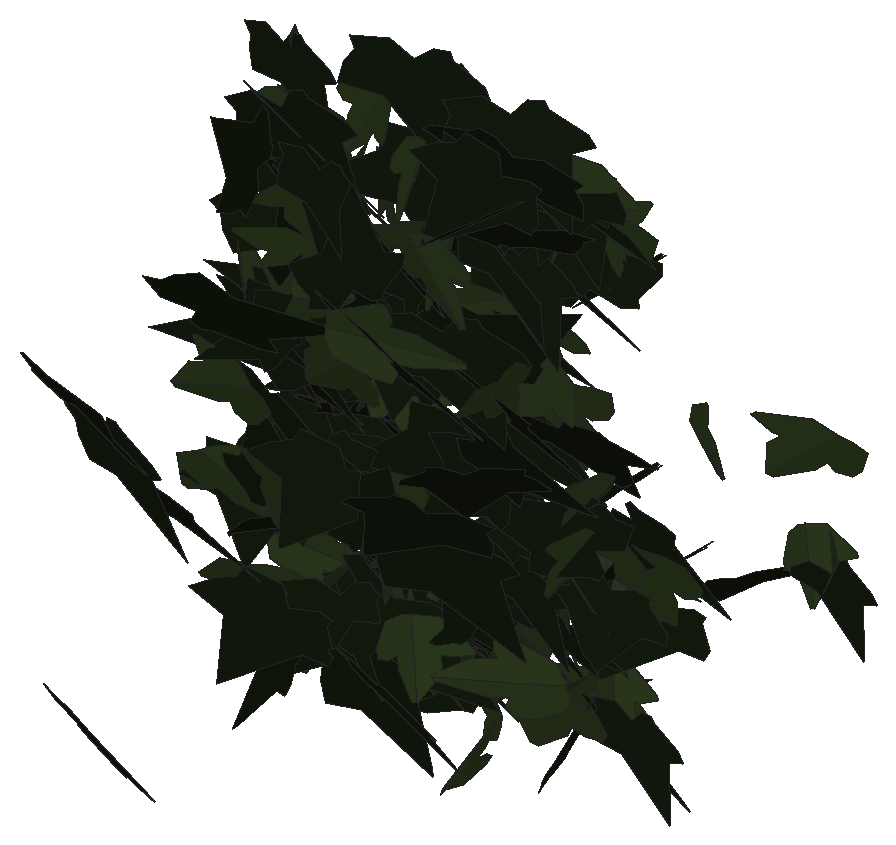
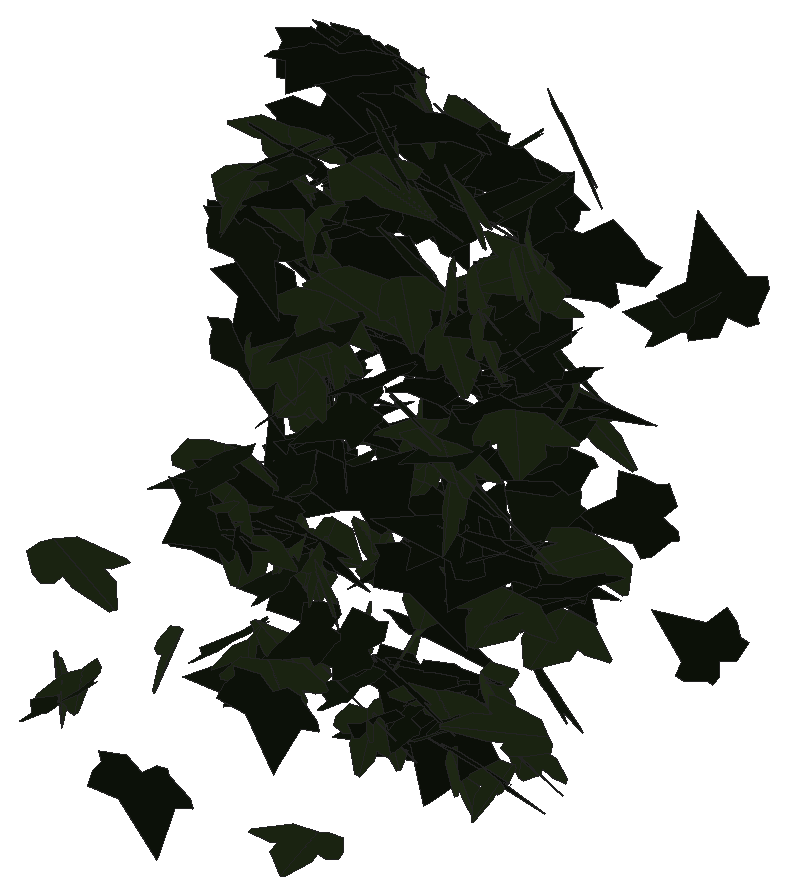
# SketchUp Ruby script. Lengths in millimetres.
U = 1.mm
M = Sketchup.active_model
def pt(a) = Geom::Point3d.new(a.map { |v| v * U })
def face(e, loops, mat)
  f = e.add_face(loops[0].map { |a| pt(a) })
  loops[1..].each { |l| e.add_face(l.map { |a| pt(a) }).erase! }
  f.material = f.back_material = mat if mat
  f
end
# faces: each face lists its corners as indices into pts; further lists are holes
def faces(e, pts, list, mat = nil) = list.each { |f| face(e, (f[0].is_a?(Array) ? f : [f]).map { |l| l.map { |i| pts[i] } }, mat) }
# xy, xz, yz: faces in a plane at the given z, y or x. An outline is a flat list of corners, or four numbers for a rectangle; further outlines are holes
def ring(l) = l.size == 4 ? [[l[0], l[1]], [l[2], l[1]], [l[2], l[3]], [l[0], l[3]]] : l.each_slice(2).to_a
def flat(e, list, mat, &to3) = list.each { |f| face(e, (f[0].is_a?(Array) ? f : [f]).map { |l| ring(l).map { |u, v| to3.(u, v) } }, mat) }
def xy(e, z, list, mat = nil) = flat(e, list, mat) { |x, y| [x, y, z] }
def xz(e, y, list, mat = nil) = flat(e, list, mat) { |x, z| [x, y, z] }
def yz(e, x, list, mat = nil) = flat(e, list, mat) { |y, z| [x, y, z] }
def lines(e, pts, list) = list.each { |a, b| e.add_line(pt(pts[a]), pt(pts[b])) }
# prism: a flat outline (further loops are holes) pulled along v
def prism(e, loops, v, mat = nil)
  f = face(e, loops, mat); d = Geom::Vector3d.new(v.map { |x| x * U })
  f.pushpull(f.normal.samedirection?(d) ? d.length : -d.length)
end
def box(e, o, s, mat = nil) = prism(e, [[o, [o[0] + s[0], o[1], o[2]], [o[0] + s[0], o[1] + s[1], o[2]], [o[0], o[1] + s[1], o[2]]]], [0, 0, s[2]], mat)
def at(x, y, z, deg = 0) = Geom::Transformation.translation(pt([x, y, z])) * Geom::Transformation.rotation(ORIGIN, Z_AXIS, deg.degrees)
def axes(o, x, y, z) = Geom::Transformation.new([*x, 0, *y, 0, *z, 0, *pt(o).to_a, 1])
def part(name) = M.definitions.add(name)
# library, detail: a bought-in or finely detailed component or shape, given as its bounding box
def library(name, o, s) = part(name).tap { |d| box(d.entities, o, s) }
def detail(e, o, s) = box(e.add_group.entities, o, s)
def put(e, d, t, mat = nil) = e.add_instance(d, t).tap { |i| i.material = mat if mat }
def group(e, t, mat = nil) = e.add_group.tap { |g| g.transformation = t; g.material = mat if mat }.entities
root = M.entities
M.materials.add("efeu1").color = [18, 25, 13]
M.materials.add("efeu2").color = [43, 57, 29]
c1 = part("ivyleaf_10")
p = [[0,12.8,-0.8],[-1.5,51.3,-10.9],[-4.9,51,-11.6],[-13.6,26.5,-7.3],[-13.2,15.9,-4.6],[-21.1,19.3,-7.2],
  [-29.5,16.3,-8.3],[-29.2,8.3,-6.2],[-19.7,-9.8,0.5],[-7.6,-13,4],[1,-12.2,5.8],[-0.4,51.1,-11.1],
  [-1.5,51.1,-10.9],[1,-12.4,5.9],[16.9,-12.4,3.5],[35.1,9.1,-5.1],[35,12.9,-6.1],[20.5,16.4,-4.9],
  [15.8,15,-3.8],[15.3,27.6,-7.1],[12.8,31.3,-7.8]]
faces(c1.entities,p,[[0,1,2,3,4,5,6,7,8,9,10],[11,12,0,13,14,15,16,17,18,19,20]],"efeu2")
c2 = part("ivyleaf_9")
p = [[39.1,54.8,31.7],[34.5,51.8,30.2],[-5.3,25.2,17.3],[-17.9,28.3,20.9],[-21.6,21.7,17],[-20.2,4.3,5.3],
  [-22.9,-0.3,2.5],[-17.1,-4,-0.6],[-2,-2.1,-1.2],[-0.7,-15.4,-10.1],[16.6,-22.3,-16.7],[21.1,-15.1,-12.5],
  [32.7,-10.7,-11],[46.1,-1.8,-6.6],[30.8,11.2,3.8]]
faces(c2.entities,p,[[0,1,2,3,4,5,6,7,8,9,10,11,12,13,14]],"efeu1")
put(root,c1,axes([5796.8,665.9,3906.6],[-0.334,1.13497,-0.54632],[0.05256,-0.548,-1.14733],[-2.39672,-0.17018,0.05097]))
put(root,c2,axes([5795.1,740.7,3667.1],[-0.39675,-1.1687,0.01594],[0.00619,-0.01677,-1.18713],[2.22447,-0.2084,0.00615]))
put(root,c2,axes([5800.6,675.8,3671.1],[-0.80713,-1.1442,0.03662],[-0.02069,-0.03502,-1.22027],[2.17866,-0.42423,0.00198]))
put(root,c2,axes([5787.4,726.4,3996.3],[0.43543,-1.15832,-0.36483],[-0.12512,0.35889,-1.18069],[2.30789,0.238,0.00482]))
put(root,c2,axes([5772.2,444.1,3486.4],[0.67007,-0.77947,0.88639],[0.78469,-0.7855,-0.85452],[2.10497,0.54095,0.03639]))
put(root,c1,axes([5771.8,776.8,3538.8],[0.44711,0.17688,1.12767],[1.75643,0.6481,-0.29392],[-1.27844,0.95227,-0.00942]))
put(root,c1,axes([5809.5,773.5,3472.8],[0.06326,0.95136,0.64808],[-0.18696,0.64833,-0.94669],[-2.18284,-0.02796,0.09987]))
put(root,c2,axes([5787.2,702.7,3951.1],[0.40232,-0.971,-0.71315],[0.22026,0.73707,-0.96926],[2.28229,0.10003,0.21925]))
put(root,c2,axes([5775.5,541.7,3704.5],[1.95629,-0.57689,0.28594],[0.45149,-0.16143,-1.17847],[1.1392,1.05464,-0.02398]))
put(root,c1,axes([5798.9,740.6,3498.4],[1.98905,-0.35637,0.40377],[0.7281,-0.12915,-1.1042],[0.7214,1.11293,0.00116]))
put(root,c1,axes([5791.5,633.5,3697],[-1.72743,-0.13985,-0.81354],[1.56922,-0.09528,-0.90351],[0.07576,-1.21515,0.16447]))
put(root,c1,axes([5857.2,580.1,3829.6],[-1.23871,0.16423,1.01664],[-1.941,0.06405,-0.66327],[-0.2719,-1.20543,0.10327]))
put(root,c1,axes([5827.5,723.1,3881.6],[-1.58643,-0.91265,0.03042],[0.20371,-0.13855,-1.22394],[1.72594,-0.82253,0.17242]))
put(root,c1,axes([5828.9,713,4076.7],[0.14606,-1.24687,-0.06836],[-0.00446,0.06835,-1.24923],[2.3766,0.07676,0.00186]))
put(root,c2,axes([5792.4,682.7,3851.4],[0.87222,-1.11921,0.29812],[0.25648,-0.2669,-1.20919],[2.18938,0.47715,0.02289]))
put(root,c1,axes([5818.1,758.2,3676.9],[-2.00969,-0.4188,-0.37007],[0.70108,0.07338,-1.13415],[0.7999,-1.11651,0.06427]))
put(root,c2,axes([5782.9,724.2,3988.2],[1.81822,-0.91922,0.37954],[0.50747,-0.27026,-1.32573],[1.82341,0.99182,-0.0095]))
put(root,c1,axes([5811.7,720.4,4118.6],[0.4129,-0.40986,1.14936],[1.34286,-0.91031,-0.45779],[1.89478,0.73446,0.07398]))
put(root,c2,axes([5854.6,731.7,3494.6],[-1.93697,0.40526,-0.37422],[0.57062,-0.25279,-1.08916],[-0.88121,-1.05449,0.11728]))
put(root,c2,axes([5807,693.3,3749.7],[0.35081,-1.06405,0.72876],[0.51452,-0.68793,-1.07282],[2.39999,0.30302,0.12347]))
put(root,c2,axes([5877.2,707.8,3857.9],[-0.54542,0.13541,1.18924],[-2.20259,-0.34334,-0.23979],[0.5812,-1.17411,0.20727]))
put(root,c2,axes([5868.5,782.2,3482.6],[-2.10767,0.22953,0.00729],[-0.07182,-0.14646,-1.12084],[-0.43113,-1.09773,0.15107]))
put(root,c2,axes([5809.5,381.8,3879.2],[2.30917,-0.69271,-0.54022],[0.98007,-0.18545,1.39436],[-1.3545,-1.31513,0.08793]))
put(root,c1,axes([5839.9,635,3591.3],[-2.1649,-0.24436,-0.30591],[0.56292,0.07954,-1.16336],[0.48823,-1.17523,-0.01513]))
put(root,c2,axes([5813.5,656.2,3828.8],[2.30353,-0.22878,0.07764],[0.14384,-0.0182,-1.23177],[0.43673,1.2127,-0.00384]))
put(root,c1,axes([5852.9,735.5,3552.3],[0.32746,-1.13453,0.29816],[0.02511,-0.29946,-1.14709],[2.23242,0.16978,-0.03083]))
put(root,c2,axes([5869.6,710.7,3988],[-1.9285,0.57898,-0.38317],[0.62719,-0.1956,-1.16703],[-1.16305,-1.06552,0.00602]))
put(root,c2,axes([5838.9,739.4,3723.2],[-0.4965,-1.17157,0.083],[0.05703,-0.09163,-1.19926],[2.23458,-0.25797,0.04905]))
put(root,c2,axes([5884.1,729.3,3790.2],[-1.72681,0.78913,0.0762],[-0.10023,0.05556,-1.20245],[-1.50552,-0.90882,-0.00735]))
put(root,c2,axes([5898.5,634.2,3865.5],[-1.72162,-0.08563,0.9191],[-1.74533,-0.06342,-0.90849],[0.20039,-1.28802,-0.01637]))
put(root,c1,axes([5859.5,785.6,3473.3],[0.10728,-1.14994,-0.01867],[-0.02692,0.01799,-1.15125],[2.18869,0.05659,-0.01325]))
put(root,c2,axes([5832.4,683.2,4146.7],[0.49684,-1.24339,0.04769],[0.00153,-0.04856,-1.27046],[2.36815,0.2609,-0.00919]))
put(root,c2,axes([5858.2,634.3,3662.5],[0.869,1.05762,0.23913],[0.22543,0.20927,-1.1517],[-2.05132,0.47103,-0.02526]))
put(root,c2,axes([5848.7,737.8,3734.2],[1.83436,0.70001,-0.10289],[-0.19701,-0.03249,-1.19071],[-1.33208,0.96876,0.03442]))
put(root,c1,axes([5820.4,705.7,4068.9],[1.68517,-0.30802,0.84232],[1.70439,0.23909,-0.85395],[0.0931,1.19848,0.38684]))
put(root,c2,axes([5827.7,716.4,4018.2],[1.91441,-0.73274,-0.00047],[0.10005,0.07297,-1.24122],[1.39096,1.00324,0.08993]))
put(root,c1,axes([5869,724.6,3991.1],[-0.11923,-1.23346,0.02125],[-0.00272,-0.0212,-1.23505],[2.34787,-0.06266,-0.00035]))
put(root,c2,axes([5872.6,629.5,3516.1],[-1.50831,0.48977,-0.69106],[1.10614,-0.374,-0.93158],[-1.17267,-0.98273,0.01012]))
put(root,c2,axes([5891.4,655.9,4009.7],[1.05856,0.02583,-1.1473],[-2.18322,-0.0237,-0.55665],[-0.06204,1.2748,0.0129]))
put(root,c2,axes([5836.2,698.7,4045.9],[1.40072,-1.00791,0.08638],[0.06612,-0.08157,-1.24786],[1.92416,0.73653,-0.02]))
put(root,c2,axes([5878.6,753.6,3737.5],[-2.02455,-0.5304,-0.16639],[0.35453,-0.00163,-1.1857],[0.99679,-1.07669,0.08376]))
put(root,c2,axes([5884.7,603.5,3706.4],[1.41341,-0.34365,0.93272],[-0.72823,0.97574,0.66417],[-1.74603,-0.68515,0.47803]))
put(root,c2,axes([5911.2,584.2,3910.9],[-1.74842,0.80914,-0.13427],[0.16788,-0.10297,-1.22405],[-1.55195,-0.92271,0.01886]))
put(root,c2,axes([5879.8,767.5,3498.2],[1.9356,0.42232,-0.42053],[-0.77024,-0.12119,-1.10048],[-0.83266,1.09384,0.04043]))
put(root,c1,axes([5892,703.1,4030.4],[-0.16776,-1.25739,-0.08719],[0.00034,0.08739,-1.26047],[2.39882,-0.08795,-0.00592]))
put(root,c1,axes([5891.6,654.6,4022],[-1.43648,-1.00158,-0.09615],[0.16857,0.05359,-1.25354],[1.90753,-0.75898,0.03837]))
put(root,c1,axes([5908.5,626.5,3973.2],[-2.07098,-0.46036,0.41268],[-0.62058,-0.28242,-1.17483],[0.99971,-1.12899,0.12561]))
put(root,c2,axes([5856,742.1,3727.9],[1.0907,-0.03688,1.05806],[1.77323,0.58893,-0.48412],[-0.95687,1.04933,0.3089]))
put(root,c1,axes([5892.9,754.6,3781.3],[0.09887,-1.02424,-0.60939],[0.21943,0.61142,-1.01784],[2.25763,-0.01457,0.12562]))
put(root,c2,axes([5859.6,646.3,3863],[1.1828,-1.04,0.1457],[0.1814,-0.11274,-1.21131],[1.9904,0.62829,0.02381]))
put(root,c2,axes([5882.4,784.9,3505.2],[-0.6573,-1.0132,0.42149],[0.09429,-0.45582,-1.05512],[2.08639,-0.2986,0.18047]))
put(root,c2,axes([5850.2,635.9,4109.5],[1.8345,-0.93429,0.32696],[0.44831,-0.22675,-1.34239],[1.82975,0.99227,0.0011]))
put(root,c2,axes([5858,378.8,3863.4],[1.06925,-1.36745,0.26542],[0.19892,-0.244,-1.47836],[2.64363,0.57144,0.00389]))
put(root,c1,axes([5894.3,771,3536.3],[2.14849,0.22971,-0.21732],[-0.39215,-0.07681,-1.15153],[-0.45653,1.14704,-0.03359]))
put(root,c2,axes([5935.6,506.4,4129.3],[-0.90013,0.22933,-1.41585],[-2.38064,0.66355,0.52532],[1.33573,1.33717,-0.01786]))
put(root,c1,axes([5881.6,1018.8,3474.9],[1.36929,0.79738,0.35485],[0.37302,0.30052,-1.07268],[-1.61863,0.7438,0.05299]))
put(root,c2,axes([5914.3,579.1,3603.7],[-2.15669,-0.46089,-0.14815],[0.25504,0.06373,-1.2233],[0.88536,-1.14106,-0.00849]))
put(root,c2,axes([5877.4,732.9,3857.4],[1.67334,-0.80287,-0.18138],[-0.19283,0.15781,-1.18969],[1.55461,0.88376,0.04766]))
put(root,c2,axes([5910.5,758,3529.7],[-1.01703,-0.93945,0.40443],[-0.30539,-0.37364,-1.07997],[1.9225,-0.55634,0.0424]))
put(root,c1,axes([5903.7,747.3,3834.8],[2.27086,-0.16716,-0.00538],[-0.0128,-0.00925,-1.20479],[0.31805,1.19315,-0.0101]))
put(root,c1,axes([5921,722.2,3955.4],[-0.74148,-1.17178,0.09335],[0.02893,-0.10336,-1.23396],[2.23702,-0.38706,0.0469]))
put(root,c2,axes([5903.8,657.5,4026.3],[-0.28963,-1.04921,0.79209],[-0.04706,-0.79495,-1.05775],[2.50155,-0.13643,0.07181]))
put(root,c2,axes([5939.1,745.7,3683.1],[0.36559,1.05919,-0.53623],[-0.37314,-0.50744,-1.07256],[-2.22844,0.25874,0.09163]))
put(root,c2,axes([5887.8,612.3,4125.7],[-0.71202,-0.29937,-1.24944],[2.25992,0.41639,-0.45532],[0.93379,-1.23599,0.14924]))
put(root,c2,axes([5939.4,744,3549.2],[-1.97214,-0.52652,0.05533],[-0.0399,-0.0807,-1.16064],[1.00681,-1.03456,0.06238]))
put(root,c1,axes([5927.4,746,3664],[-2.18693,-0.30642,-0.11692],[0.2528,-0.04533,-1.1867],[0.57069,-1.15412,0.07765]))
put(root,c2,axes([5875.3,501.7,3952.1],[0.53463,-0.35415,1.26589],[2.33503,-0.39399,-0.38248],[0.89796,1.23538,0.24091]))
put(root,c2,axes([5900.3,747.1,3521.8],[1.42691,-0.88297,0.03543],[0.01785,-0.03851,-1.1582],[1.68172,0.74959,-0.01777]))
put(root,c1,axes([5951.2,535,3772.4],[-1.98349,0.48543,0.45725],[-0.82928,0.14655,-1.14871],[-0.96081,-1.12861,0.04751]))
put(root,c1,axes([5935.5,687.1,4122.8],[1.54118,-0.96446,-0.08158],[-0.10404,0.06063,-1.25934],[1.83918,0.81162,-0.00288]))
put(root,c2,axes([5959.9,730.9,3688.7],[-1.55565,-0.63087,0.84082],[-1.25444,-0.52211,-1.0325],[1.55846,-1.05,0.00822]))
put(root,c2,axes([5918.9,735.8,3736.1],[1.98078,-0.36395,-0.46289],[-0.8344,0.14857,-1.10256],[0.74811,1.12933,-0.00413]))
put(root,c1,axes([5926.5,713.4,4026.2],[0.89529,-1.13561,-0.10487],[0.67342,0.25318,-1.15439],[2.06339,0.41011,0.42225]))
put(root,c2,axes([5974.4,776.5,3458.2],[-0.5602,-0.0008,1.12445],[-2.04946,-0.33441,-0.28213],[0.61608,-1.11319,0.08394]))
put(root,c2,axes([5902.7,641.9,3924.4],[0.48464,-0.04985,1.34194],[2.46138,0.37684,-0.23141],[-0.68809,1.31288,0.11738]))
put(root,c2,axes([5970.4,778.5,3552.3],[-2.02836,0.4474,-0.10971],[0.21814,-0.01027,-1.15534],[-0.84915,-1.07135,-0.03474]))
put(root,c2,axes([5974.5,711.9,3579.9],[-2.1723,-0.06918,0.19169],[-0.36733,0.0169,-1.14314],[0.1245,-1.15725,-0.02815]))
put(root,c2,axes([5946.2,742.1,3535],[1.82326,0.53116,-0.38862],[-0.87864,0.05321,-1.06534],[-0.89273,1.03245,0.25484]))
put(root,c1,axes([5940.6,571,3961.2],[0.00175,-0.48505,-1.13365],[0.82398,1.0616,-0.45388],[2.19734,-0.3977,0.1711]))
put(root,c2,axes([5935.9,639.5,3595.8],[-0.39883,-1.09969,-0.5919],[0.3071,0.5713,-1.11855],[2.35692,-0.26052,0.04559]))
put(root,c2,axes([5989.9,717.6,3842.9],[-1.94961,0.67503,-0.19723],[0.28481,-0.13126,-1.2265],[-1.30777,-1.03491,0.02691]))
put(root,c2,axes([5933.5,781.9,3502],[1.53642,-0.8004,-0.01432],[0.00238,0.02159,-1.1367],[1.52357,0.80712,0.01621]))
put(root,c2,axes([5961.1,696.5,3879.7],[-0.92994,-1.08793,-0.09546],[0.09798,0.08152,-1.19254],[2.07619,-0.49114,0.01352]))
put(root,c1,axes([5974.8,766.5,3488.4],[-0.45545,-1.15253,-0.03923],[0.02595,0.03724,-1.1771],[2.19462,-0.23963,0.00578]))
put(root,c2,axes([5939.7,646.9,3675.7],[0.34383,-0.8034,1.01493],[0.46614,-0.98504,-0.82334],[2.41904,0.30401,0.0144]))
put(root,c1,axes([6004.9,554.6,3915.9],[-1.73918,0.26509,0.79226],[-1.43493,0.24408,-0.95131],[-0.68488,-1.18455,-0.01872]))
put(root,c1,axes([5983.8,790.7,3481.1],[-1.68336,0.68941,0.18401],[-0.31963,0.0837,-1.12083],[-1.31987,-0.89954,0.03674]))
put(root,c1,axes([5986.6,719.4,3989.9],[-0.77755,-1.17096,-0.06937],[0.05362,0.06364,-1.24017],[2.23183,-0.40948,0.00563]))
put(root,c2,axes([5961,583.6,3785.6],[0.08989,-0.99937,-0.91828],[-0.11716,0.91631,-1.0004],[2.58036,0.07642,-0.01343]))
put(root,c1,axes([5969.5,695,3817.3],[1.12076,1.07279,0.10328],[0.09382,0.09076,-1.22379],[-2.04902,0.59094,0.00046]))
put(root,c1,axes([5983.9,699,3556.6],[0.52306,-0.30312,-1.14992],[0.24851,1.18078,-0.28005],[2.2496,-0.05996,0.29831]))
put(root,c2,axes([5966.1,569.1,4105],[0.21019,-1.23066,0.15811],[-0.01356,-0.15936,-1.23542],[2.36141,0.10862,-0.02117]))
put(root,c2,axes([5969.2,656.5,3688.8],[0.89681,-0.53052,-1.0117],[-0.46102,1.0231,-0.64932],[2.12471,0.44592,0.28614]))
put(root,c2,axes([5968.7,712.9,3911],[-1.12934,-0.69771,-0.81354],[1.63779,0.24412,-0.83704],[1.21584,-0.97692,0.37186]))
put(root,c1,axes([5985.4,659,3605.1],[-0.27073,0.89512,-0.75729],[0.10158,-0.75711,-0.90493],[-2.22916,-0.14321,0.05073]))
put(root,c2,axes([6040.5,651.3,4092.1],[-2.08319,0.48971,0.33079],[-0.73068,-0.05992,-1.18167],[-0.85505,-1.14189,0.20387]))
put(root,c2,axes([6012.2,545,3803.8],[-1.89197,-0.72797,-0.00491],[0.00718,0.00316,-1.23214],[1.38548,-0.99411,-0.00033]))
put(root,c2,axes([6031.1,776.6,3508.2],[-1.8215,0.61294,-0.09726],[0.17801,-0.03425,-1.13632],[-1.16765,-0.96139,-0.02152]))
put(root,c1,axes([5999.3,688.9,3721.3],[-2.03344,-0.33034,-0.38585],[0.78882,-0.04749,-1.10703],[0.55884,-1.13498,0.15862]))
put(root,c2,axes([6025.5,747.8,3721.1],[1.41391,-0.51743,0.79441],[-1.25713,0.44148,0.90527],[-1.29433,-0.99403,-0.01146]))
put(root,c2,axes([5997.1,673.4,4191.4],[-1.35894,-0.64221,-0.79349],[1.36033,0.37683,-0.94817],[1.3871,-0.99873,0.15248]))
put(root,c2,axes([6053.6,644.2,3991.5],[-1.5359,0.93613,0.24763],[-0.37252,0.158,-1.23517],[-1.80488,-0.82923,0.04421]))
put(root,c2,axes([5996.8,789.8,3523.6],[0.47054,-1.0883,0.22054],[0.19352,-0.2028,-1.11477],[2.10448,0.26198,0.0532]))
put(root,c2,axes([6055.6,524.2,3772.9],[-0.07097,0.4332,1.25952],[-0.82498,1.18747,-0.42125],[-2.39694,-0.42153,0.10769]))
put(root,c1,axes([6048.4,712.9,4116.5],[1.31907,0.56764,-0.87375],[-1.64029,-0.2774,-0.86386],[-1.11439,1.08021,0.2373]))
put(root,c2,axes([6031.1,611.9,4003.9],[1.37632,-1.07781,0.32059],[-0.21149,0.3108,1.29555],[-2.12963,-0.72742,0.07853]))
put(root,c2,axes([6038.5,697,4158.1],[-1.57234,0.55261,-0.75821],[1.22708,-0.39953,-0.99372],[-1.2972,-1.04775,-0.02098]))
put(root,c2,axes([5999.2,776.2,3564.8],[1.37643,-0.87902,0.24827],[0.40418,-0.14617,-1.13617],[1.69075,0.75054,0.06949]))
put(root,c2,axes([6023.4,727.7,3875],[-0.37138,-1.19943,0.01731],[-0.02021,-0.01581,-1.21518],[2.28291,-0.19526,-0.00794]))
put(root,c2,axes([6063.5,496.4,4048.1],[-1.99499,0.78346,-0.45317],[-0.689,0.27258,1.30866],[1.57876,1.10898,-0.00151]))
put(root,c2,axes([5994.1,577.7,3737.3],[2.16241,-0.15173,0.67227],[1.2595,-0.12169,-1.14593],[0.36618,1.31457,-0.02849]))
put(root,c2,axes([6081.6,668.1,3785.5],[-0.57598,0.68352,0.93082],[-1.00981,0.77237,-0.73968],[-1.95215,-0.6012,0.10799]))
put(root,c2,axes([6086.8,684,4102.4],[-2.05599,0.51894,0.31171],[-0.57094,0.09493,-1.19769],[-1.00071,-1.12034,0.0429]))
put(root,c2,axes([6085.4,617.8,3822.8],[-1.86236,0.66687,0.18267],[-0.30729,0.08741,-1.18403],[-1.27956,-0.9916,0.01848]))
put(root,c2,axes([6026,594.1,3616.6],[0.93251,-0.71755,-1.15566],[-0.30267,1.1897,-0.80611],[2.57117,0.40029,0.32424]))
put(root,c2,axes([6027.2,564.9,3584.4],[-0.85472,-0.2473,-1.12295],[2.05271,0.32732,-0.50343],[0.75863,-1.16429,0.09699]))
put(root,c1,axes([6067.2,656.6,3674.8],[-1.56945,0.76915,0.3218],[-0.45142,0.21749,-1.12766],[-1.52124,-0.85807,0.00263]))
put(root,c1,axes([6092.4,701.7,3952.5],[1.30962,0.32757,-0.9884],[-1.96323,0.05294,-0.70061],[-0.27017,1.20317,0.29993]))
put(root,c1,axes([6070.1,1022.6,3658.1],[-0.95019,0.95392,0.44885],[-0.34547,0.41144,-1.07632],[-1.97647,-0.53052,-0.02766]))
put(root,c1,axes([6064,589.9,4150.1],[1.163,-0.96069,0.51278],[0.52802,-0.43124,-1.13857],[2.00415,0.67111,0.00241]))
put(root,c1,axes([6068.9,703.1,3495.3],[-1.01131,0.89456,0.65066],[0.60354,-0.56835,1.04037],[2.01688,0.61863,0.01493]))
put(root,c1,axes([6079.3,753.9,3625],[0.98036,-1.02657,-0.21563],[-0.13615,0.20529,-1.14823],[1.99176,0.51932,0.02765]))
put(root,c1,axes([6076.2,564,3739.3],[0.15864,-1.21645,0.30468],[0.22518,-0.29636,-1.21561],[2.37601,0.1093,0.09486]))
put(root,c2,axes([6053.1,773.1,3569.3],[1.61064,-0.74689,-0.2137],[-0.33669,0.12243,-1.12846],[1.43967,0.86422,-0.02483]))
put(root,c2,axes([6050.8,706.5,3816.8],[1.79573,-0.81452,-0.23788],[-0.31949,0.16953,-1.24634],[1.58303,0.95818,0.0183]))
put(root,c2,axes([6091.5,1050.2,3493.5],[0.47299,1.10795,-0.11448],[-0.1735,-0.09667,-1.13347],[-2.11276,0.25598,0.06745]))
put(root,c1,axes([6089.6,739.9,3638.5],[-0.49991,1.10482,0.38543],[-0.47999,0.33228,-1.12435],[-2.17463,-0.32732,0.15957]))
put(root,c1,axes([6091,722.3,3899.2],[1.78325,-0.7882,-0.09332],[0.13848,0.22907,-1.20421],[1.50421,0.91332,0.22149]))
put(root,c2,axes([6104,805.2,3483.3],[0.56342,1.10278,0.04301],[-0.00566,0.04532,-1.14173],[-2.1004,0.29569,0.01461]))
put(root,c2,axes([6081.7,714,3725.2],[-0.10336,0.44264,1.33266],[-0.2745,-1.32836,0.43534],[2.65844,-0.11995,0.09676]))
put(root,c1,axes([6088.3,603.1,4056.1],[1.23356,-0.97045,0.48091],[0.5425,-0.38785,-1.16682],[1.98863,0.70778,0.02]))
put(root,c1,axes([6098.8,718.4,3927.9],[-2.27533,0.13285,-0.14595],[0.26178,-0.08177,-1.2011],[-0.26937,-1.20163,0.0656]))
put(root,c2,axes([6081.9,708.9,3927.9],[1.91378,-0.444,-0.55518],[-0.70738,0.49145,-1.06623],[1.1533,1.0382,0.26729]))
put(root,c1,axes([6097.2,549.9,3655.6],[0.97862,1.12279,-0.18676],[-0.14552,-0.17039,-1.23493],[-2.16137,0.51985,-0.00141]))
put(root,c1,axes([6114.3,658.9,3793.7],[0.27969,-0.72313,-0.979],[-0.2398,0.97177,-0.7367],[2.30395,0.18893,0.04217]))
put(root,c2,axes([6092.4,677.9,4125.1],[-0.42243,-1.22239,0.01612],[-0.0033,-0.01607,-1.24238],[2.32666,-0.22196,0.00117]))
put(root,c2,axes([6133.7,746.8,3657.6],[-2.23755,0.08003,-0.01328],[0.02518,-0.00121,-1.1784],[-0.15233,-1.17575,0.00031]))
put(root,c2,axes([6086.1,721.5,3723],[-0.0457,-1.1326,0.44618],[0.28741,-0.44559,-1.12298],[2.29891,0.0332,0.14927]))
put(root,c1,axes([6114.6,790,3501.7],[1.89902,0.50477,-0.25471],[-0.69216,0.17741,-1.07311],[-0.82392,1.01441,0.31442]))
put(root,c2,axes([6072.1,528.1,3595.3],[0.79393,-1.00323,0.78821],[0.88491,-0.6527,-1.07683],[2.26117,0.60768,0.14467]))
put(root,c1,axes([6103.8,753,3487.5],[-0.42973,-1.13162,0.41676],[0.54374,0.36173,1.137],[-2.22978,0.3063,0.19694]))
put(root,c1,axes([6116.5,715.5,4023.4],[-0.04316,-0.9765,0.74349],[0.69365,-0.71543,-0.92853],[2.23047,0.20359,0.30315]))
put(root,c1,axes([6124.6,741,3656.2],[-1.3214,0.94249,0.13022],[-0.09304,0.12565,-1.1701],[-1.80839,-0.69515,-0.03495]))
put(root,c1,axes([6120.9,730.1,3840.4],[-1.81486,0.71123,-0.27459],[0.3724,-0.19668,-1.18895],[-1.40238,-0.97264,0.03963]))
put(root,c2,axes([6108.7,646.3,3694.1],[-0.01279,-0.69302,-1.08896],[0.0599,1.08856,-0.69296],[2.45588,-0.03016,0.01123]))
put(root,c2,axes([6134.5,612.9,3814.3],[-0.76936,-0.74245,0.89804],[-0.79987,-0.79367,-0.84533],[2.06835,-0.58309,0.00714]))
put(root,c1,axes([6143.3,729.2,3854],[-1.5297,-0.85619,0.34099],[-0.30802,-0.31429,-1.17063],[1.72672,-0.81456,0.09326]))
put(root,c2,axes([6104.1,778.1,3618.2],[0.77975,-1.08647,0.0558],[0.0233,-0.05502,-1.16113],[2.07036,0.40981,-0.00795]))
put(root,c1,axes([6128.1,669,3615.3],[-0.41808,-0.9108,-0.79876],[0.52457,0.75292,-0.93433],[2.24513,-0.34552,0.06956]))
put(root,c2,axes([6114,649.8,3692.9],[1.91054,0.61352,0.20599],[0.27295,0.15982,-1.17493],[-1.20109,1.01223,0.06066]))
put(root,c2,axes([6084.6,477.4,4012.3],[1.49461,-0.97461,0.83994],[1.07165,-0.62446,-1.25104],[2.20173,0.96554,0.03873]))
put(root,c2,axes([6118.1,691.1,3826.7],[1.07179,-0.72783,-0.80416],[-0.55086,0.77239,-0.90177],[1.98941,0.60599,0.18354]))
put(root,c1,axes([6121.3,533.1,4088.6],[-1.53731,0.54525,-0.78349],[0.89503,-0.66584,-0.94821],[-1.5809,-0.90718,0.22505]))
put(root,c2,axes([6105.1,626.9,3933.3],[-0.71844,-0.04199,1.26437],[2.3327,-0.33884,0.35469],[0.59614,1.27527,0.13587]))
put(root,c1,axes([6103.5,449.7,4026.3],[0.02648,0.03971,1.26397],[1.89655,0.77789,-0.03541],[-1.48177,0.99634,-0.02273]))
put(root,c2,axes([6174.8,762.7,3643.5],[-2.02883,-0.31545,0.39903],[-0.72918,-0.11152,-1.1117],[0.63677,-1.13277,-0.00168]))
put(root,c2,axes([6171.8,552.4,3694.2],[-0.23016,1.05167,0.71168],[-0.33015,0.69452,-1.05579],[-2.39411,-0.19688,0.07717]))
put(root,c2,axes([6171.6,604.1,4178.3],[1.30511,0.53888,-1.11801],[-1.80685,-0.59496,-0.86908],[-1.52142,1.16885,0.07307]))
put(root,c2,axes([6154.4,650.6,3730.7],[0.3503,-0.85984,-1.05865],[0.4113,-1.03636,0.87931],[-2.56287,-0.28384,-0.00358]))
put(root,c2,axes([6126.4,556.9,3987.9],[-1.04461,-0.74019,-0.97444],[1.12034,0.77657,-0.92146],[2.04175,-0.80482,0.00707]))
put(root,c2,axes([6131,635.8,4062.1],[0.33563,-1.26022,-0.02444],[-0.01014,0.02393,-1.2725],[2.39888,0.17642,-0.00196]))
put(root,c2,axes([6187,613.2,4100],[0.05751,0.95124,-0.8139],[-0.98147,-0.7324,-0.87513],[-2.17111,0.35628,0.37405]))
put(root,c1,axes([6151.9,548.2,3517.5],[0.41172,-1.16598,0.38725],[-0.00465,0.3928,1.18405],[-2.33829,-0.20608,0.06583]))
put(root,c1,axes([6156.5,785.4,3519.8],[0.34556,1.07975,-0.35314],[-0.15142,-0.34466,-1.09473],[-2.15679,0.1972,0.02028]))
put(root,c1,axes([6166.8,684,4075.1],[1.05147,-1.11838,-0.16451],[-0.07476,0.164,-1.24685],[2.15011,0.55263,0.0371]))
put(root,c2,axes([6181,571.2,4174.3],[-2.34142,-0.13136,-0.22513],[0.42547,0.02671,-1.23724],[0.25507,-1.2504,-0.00278]))
put(root,c2,axes([6123.4,702.5,4011.3],[1.28944,-0.9239,0.43684],[0.72924,-0.25623,-1.1362],[1.80312,0.76432,0.14713]))
put(root,c2,axes([6179.7,535.4,4140.8],[0.21994,1.30987,0.14498],[0.0243,0.14441,-1.31496],[-2.50804,0.11627,-0.00003]))
put(root,c2,axes([6165.5,709,4108.5],[-2.03309,-0.32178,-0.57465],[1.18851,-0.14693,-1.07859],[0.3983,-1.20407,0.2852]))
put(root,c2,axes([6131.2,714.8,4102],[1.44803,-0.96644,-0.22548],[0.16648,0.34832,-1.19781],[1.88137,0.71301,0.27953]))
put(root,c2,axes([6145.5,638.1,4196.9],[-0.61751,-1.05969,-0.76898],[0.65243,0.69585,-1.10355],[2.40493,-0.46087,0.10193]))
put(root,c1,axes([6197.5,726.2,4060.1],[-1.79333,-0.36306,0.71281],[-1.1564,-0.39157,-1.00264],[0.99027,-1.11474,0.12003]))
put(root,c2,axes([6183.6,706.5,4000.1],[-2.43271,-0.28751,0.55165],[1.02646,0.116,1.31015],[-0.58999,1.38734,0.00478]))
put(root,c1,axes([6175.1,762.7,3639.8],[-2.24275,0.07851,0.02241],[-0.04248,0.00209,-1.18102],[-0.14946,-1.17862,-0.0006]))
put(root,c1,axes([6162.2,700.4,4118],[2.3067,0.29471,0.06526],[0.09798,0.06428,-1.24631],[-0.56606,1.21206,0.05023]))
put(root,c2,axes([6154.4,638.4,4045.8],[0.10965,-1.28584,-0.10032],[-0.00779,0.10024,-1.28713],[2.45463,0.05776,0.0004]))
put(root,c1,axes([6195.6,641.7,3570.8],[-2.09033,-0.17416,0.35895],[-0.66847,-0.0766,-1.11187],[0.36017,-1.15295,0.01965]))
put(root,c1,axes([6185,637.3,3931.8],[1.94429,-0.59653,-0.373],[-0.57121,0.22528,-1.18228],[1.21103,1.06397,0.0412]))
put(root,c2,axes([6159.6,709.5,4101],[-0.0723,-1.25343,-0.06295],[-0.00368,0.06304,-1.254],[2.38853,-0.03785,-0.00384]))
put(root,c2,axes([6174.2,764.2,3654.5],[-0.55124,0.22164,-1.12381],[1.34482,-0.87777,-0.35523],[-1.71581,-0.75918,0.08263]))
put(root,c2,axes([6147.5,782.1,3481.8],[1.23879,-0.93631,0.19432],[0.24716,-0.14634,-1.1401],[1.8031,0.66333,0.02277]))
put(root,c1,axes([6192.6,663.8,3654.3],[-0.77171,0.94822,0.55284],[-0.84615,0.39695,-1.00694],[-1.90993,-0.55899,0.22273]))
put(root,c1,axes([6168,754.2,3665.8],[1.53792,0.82571,0.10135],[0.17348,0.05255,-1.15498],[-1.57375,0.8127,-0.02828]))
put(root,c2,axes([6205,734.4,4000.9],[-0.33979,1.21356,0.01299],[-0.00586,0.01267,-1.22662],[-2.30976,-0.17856,0.0012]))
put(root,c2,axes([6165.6,706,3672],[-0.24348,-0.43461,1.20596],[0.34818,-1.20573,-0.41512],[2.4147,0.13003,0.18146]))
put(root,c2,axes([6160.6,744.1,3686.5],[2.21192,0.16587,0.15595],[0.24369,0.19452,-1.16118],[-0.35827,1.15638,0.17296]))
put(root,c2,axes([6194.6,507.4,3880.8],[1.15588,1.05679,-0.31651],[-0.2812,-0.28013,-1.21883],[-2.08064,0.62495,-0.01111]))
put(root,c2,axes([6246.3,629.2,3766.5],[-1.10503,0.49092,0.97923],[-1.90576,0.21142,-0.69972],[-0.84514,-1.11862,0.2975]))
put(root,c1,axes([6193,1034.7,3576.6],[0.52009,1.14546,-0.19753],[-0.1524,-0.18388,-1.1771],[-2.20697,0.28263,0.03473]))
put(root,c2,axes([6158.5,560.4,3943.1],[2.34152,-0.61089,0.13596],[0.22945,-0.06292,-1.37362],[1.16878,1.23619,-0.00272]))
put(root,c2,axes([6202,633.9,3508.6],[0.30003,0.44256,1.24519],[0.66108,1.19605,-0.46907],[-2.42664,0.38055,0.02617]))
put(root,c1,axes([6227.2,1014.5,3707],[-1.6433,-0.46477,0.66975],[-0.99641,-0.43167,-0.97451],[1.18928,-1.00387,0.10896]))
put(root,c2,axes([6168.7,490.7,3799.7],[-0.89658,-0.31019,-1.2433],[1.92892,0.72037,-0.56374],[1.49229,-1.1175,-0.0183]))
put(root,c1,axes([6201.6,729.5,4056.1],[-0.11736,1.04487,0.65522],[-0.3129,0.64321,-1.04121],[-2.32629,-0.13923,0.10699]))
put(root,c2,axes([6153.5,579.9,3869.1],[1.10575,-0.096,-1.12494],[2.1314,0.20958,0.56051],[0.27273,-1.24865,0.18057]))
put(root,c2,axes([6217.1,776.6,3624.6],[-1.87822,-0.60213,-0.04896],[0.0713,0.0326,-1.15603],[1.14754,-0.98755,-0.00831]))
put(root,c1,axes([6207.4,540.6,3969.4],[-0.58463,-1.06897,-0.57591],[0.31944,0.55097,-1.1122],[2.28875,-0.34995,0.00812]))
put(root,c2,axes([6193.2,624.6,3676.6],[1.96377,-0.26269,-0.64957],[-0.90737,0.58411,-0.99354],[0.97723,1.07024,0.38281]))
put(root,c1,axes([6207.2,764.2,3677.7],[-1.93823,0.50851,-0.21546],[0.31887,-0.14621,-1.13697],[-1.00156,-1.03063,0.05499]))
put(root,c2,axes([6206.8,775,3655.9],[0.85636,0.54735,0.92162],[0.62869,0.88007,-0.68395],[-1.94075,0.52661,0.1851]))
put(root,c2,axes([6187.7,591,3739.9],[0.53717,-1.20095,0.23748],[0.20694,-0.21815,-1.23245],[2.3207,0.29744,0.05493]))
put(root,c2,axes([6237.1,389.9,3903.8],[0.90661,0.77697,-0.89756],[-1.10347,-0.69166,-0.90645],[-1.97157,0.74441,0.0946]))
put(root,c1,axes([6255.5,540.5,3660.1],[-0.67018,0.14807,1.18152],[-1.73143,-0.82841,-0.16732],[1.4622,-0.91308,0.3434]))
put(root,c1,axes([6227.1,1023.8,3568.3],[0.35305,-0.83102,-0.84],[-0.20885,0.83449,-0.84981],[2.23911,0.20887,0.05318]))
put(root,c2,axes([6197.1,758.8,3498.2],[0.22702,-1.17597,0.11698],[0.07173,-0.11373,-1.18172],[2.24801,0.12239,0.02589]))
put(root,c1,axes([6233.2,733,3702.5],[-2.23773,-0.05594,0.1598],[-0.3013,-0.03425,-1.1768],[0.11424,-1.18609,0.02644]))
put(root,c1,axes([6230.4,667.6,3810.8],[0.0686,-1.07618,0.63458],[-0.00578,-0.63492,-1.07658],[2.37774,0.02951,-0.02093]))
put(root,c2,axes([6208.2,638.4,3876.2],[2.29183,0.31475,-0.16015],[-0.29313,-0.04406,-1.24465],[-0.60484,1.214,-0.00365]))
put(root,c2,axes([6204.6,1048.3,3547.8],[0.21704,-1.1227,0.22085],[0.1315,-0.21478,-1.12754],[2.1737,0.12509,0.04616]))
put(root,c2,axes([6198.4,762.8,3716.2],[1.3449,-0.92144,-0.233],[0.04963,0.30903,-1.14303],[1.8082,0.67687,0.20467]))
put(root,c2,axes([6251.8,668.4,3814.4],[-0.34995,1.24997,0.05276],[-0.02958,0.05104,-1.2634],[-2.38088,-0.18436,0.00794]))
put(root,c1,axes([6234.2,636,3761.6],[0.07942,-1.01204,0.7265],[0.14292,-0.72354,-1.01224],[2.36671,0.07765,0.03675]))
put(root,c2,axes([6224.3,689.7,3681.8],[-1.09426,-1.04397,0.24353],[0.29327,-0.35396,-1.15357],[2.01904,-0.51439,0.29954]))
